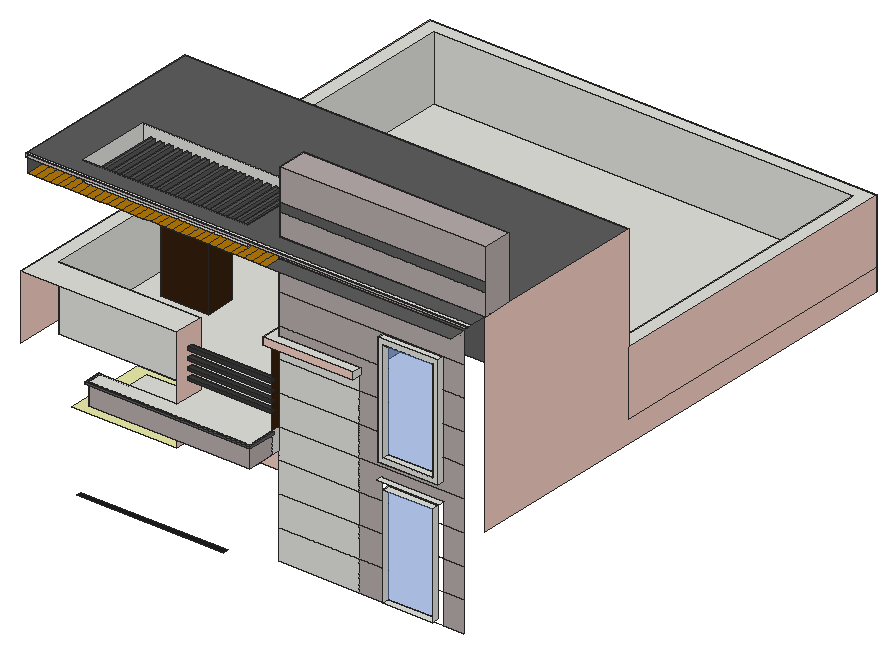
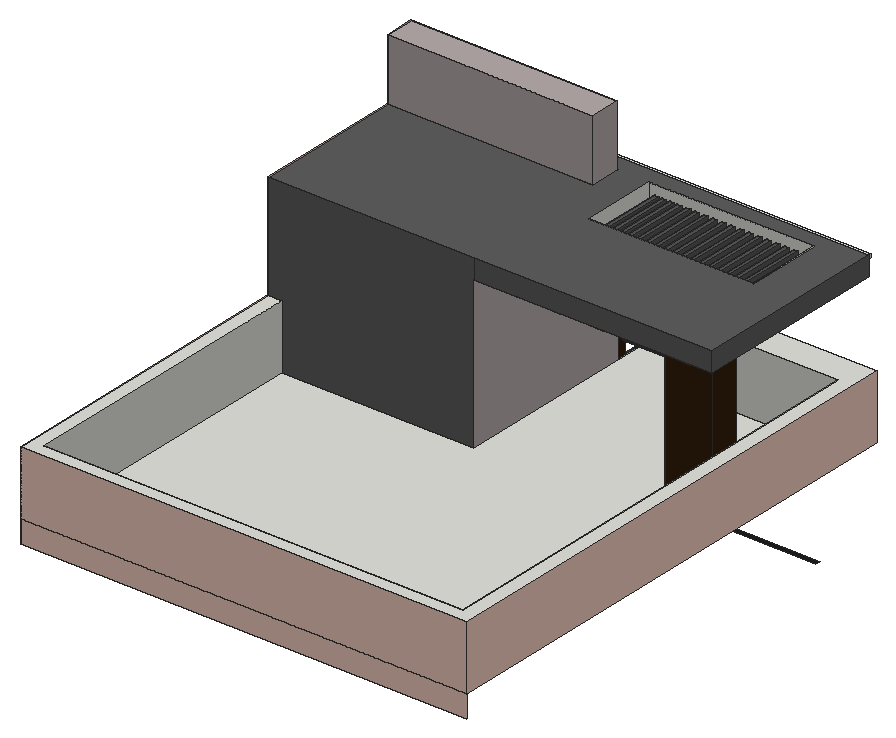
# SketchUp Ruby script. Lengths in inches.
U = 1.inch
M = Sketchup.active_model
def pt(a) = Geom::Point3d.new(a.map { |v| v * U })
def face(e, loops, mat)
  f = e.add_face(loops[0].map { |a| pt(a) })
  loops[1..].each { |l| e.add_face(l.map { |a| pt(a) }).erase! }
  f.material = f.back_material = mat if mat
  f
end
# faces: each face lists its corners as indices into pts; further lists are holes
def faces(e, pts, list, mat = nil) = list.each { |f| face(e, (f[0].is_a?(Array) ? f : [f]).map { |l| l.map { |i| pts[i] } }, mat) }
# xy, xz, yz: faces in a plane at the given z, y or x. An outline is a flat list of corners, or four numbers for a rectangle; further outlines are holes
def ring(l) = l.size == 4 ? [[l[0], l[1]], [l[2], l[1]], [l[2], l[3]], [l[0], l[3]]] : l.each_slice(2).to_a
def flat(e, list, mat, &to3) = list.each { |f| face(e, (f[0].is_a?(Array) ? f : [f]).map { |l| ring(l).map { |u, v| to3.(u, v) } }, mat) }
def xy(e, z, list, mat = nil) = flat(e, list, mat) { |x, y| [x, y, z] }
def xz(e, y, list, mat = nil) = flat(e, list, mat) { |x, z| [x, y, z] }
def yz(e, x, list, mat = nil) = flat(e, list, mat) { |y, z| [x, y, z] }
def lines(e, pts, list) = list.each { |a, b| e.add_line(pt(pts[a]), pt(pts[b])) }
# prism: a flat outline (further loops are holes) pulled along v
def prism(e, loops, v, mat = nil)
  f = face(e, loops, mat); d = Geom::Vector3d.new(v.map { |x| x * U })
  f.pushpull(f.normal.samedirection?(d) ? d.length : -d.length)
end
def box(e, o, s, mat = nil) = prism(e, [[o, [o[0] + s[0], o[1], o[2]], [o[0] + s[0], o[1] + s[1], o[2]], [o[0], o[1] + s[1], o[2]]]], [0, 0, s[2]], mat)
def at(x, y, z, deg = 0) = Geom::Transformation.translation(pt([x, y, z])) * Geom::Transformation.rotation(ORIGIN, Z_AXIS, deg.degrees)
def axes(o, x, y, z) = Geom::Transformation.new([*x, 0, *y, 0, *z, 0, *pt(o).to_a, 1])
def part(name) = M.definitions.add(name)
# library, detail: a bought-in or finely detailed component or shape, given as its bounding box
def library(name, o, s) = part(name).tap { |d| box(d.entities, o, s) }
def detail(e, o, s) = box(e.add_group.entities, o, s)
def put(e, d, t, mat = nil) = e.add_instance(d, t).tap { |i| i.material = mat if mat }
def group(e, t, mat = nil) = e.add_group.tap { |g| g.transformation = t; g.material = mat if mat }.entities
root = M.entities
M.materials.add("Generic").color = [94, 94, 94]
M.materials.add("Generic\#1").color = [182, 171, 171]
M.materials.add("Generic\#4").color = [178, 120, 8]
M.materials.add("Generic\#5").color = [242, 205, 193]
M.materials.add("Generic\#7").color = [235, 237, 171]
M.materials.add("[Color M06]").color = [86, 86, 86]
M.materials.add("[Color M07]").color = [58, 58, 58]
M.materials.add("[Color M08]").color = [30, 30, 30]
M.materials.add("[Translucent Glass Blue]").color = [100, 149, 237]
M.materials["[Translucent Glass Blue]"].alpha = 0.5
M.materials.add("[Wood Floor Dark]").color = [53, 32, 13]
xy(root,173.625,[[43.84,66.48,170.12,70.85]],"[Color M08]")
xy(root,177.11,[[299.95,74.6,342.64,79.98]])
xy(root,217.95,[[81.41,131.85,161.72,167.54]])
xy(root,243.9375,[[43.84,60.73,133.85,79.98],[43.84,79.98,206.39,131.85]],"Generic\#7")
xy(root,258.75,[[170.12,61.18,206.39,72.04]])
xy(root,258.75,[[68.34,48.23,68.34,60.73,133.85,60.73,170.12,61.18,206.39,61.18,206.39,48.23]],"Generic\#1")
xy(root,258.75,[[133.85,60.73,133.85,79.98,206.39,79.98,206.39,72.04,170.12,72.04,170.12,61.18]],"Generic\#5")
xy(root,264.3,[[299.95,74.6,342.64,79.98]])
xy(root,269.6,[[294.65,74.6,347.95,79.98]])
xy(root,275.5,[[66.59,46.29,66.59,61.66,68.34,61.66,68.34,48.23,206.39,48.23,206.39,71.98,208.2,71.98,208.2,46.29]],"Generic")
xy(root,277.5,[[[68.34,48.23,206.39,48.23,206.39,234.29,371.3125,234.29,371.3125,488.54,12.4375,488.54,12.4375,86.6,133.91,86.6,133.91,60.73,68.34,60.73],[32.8,169.87,74.12,194.99]],[93.09,60.73,133.91,79.98]])
xy(root,277.5,[[66.59,46.29,208.2,46.29,208.2,71.98,206.39,71.98,206.39,48.23,68.34,48.23,68.34,61.66,66.59,61.66]],"Generic")
xy(root,284.35,[[295.76,74.6,346.84,79.98]])
xy(root,288.55,[[299.95,74.6,342.64,79.98]])
xy(root,290.9,[[133.91,72.1,206.39,75.91]],"[Color M07]")
xy(root,293.86,[[133.91,72.1,206.39,75.91]],"[Color M07]")
xy(root,298.59,[[133.91,72.1,206.39,75.91]],"[Color M07]")
xy(root,301.54,[[133.91,72.1,206.39,75.91]],"[Color M07]")
xy(root,306.28,[[133.91,72.1,206.39,75.91]],"[Color M07]")
xy(root,309.23,[[133.91,72.1,206.39,75.91]],"[Color M07]")
xy(root,313.96,[[133.91,72.1,206.39,75.91]],"[Color M07]")
xy(root,317.11,[[133.91,72.1,206.39,75.91]],"[Color M07]")
xy(root,332.8125,[[0,60.73,133.91,60.73,133.91,86.6,12.4375,86.6,12.4375,488.54,371.3125,488.54,371.3125,234.29,382.6875,234.29,382.6875,499.98,0,499.98]])
xy(root,341.34,[[199.14,71.98,206.39,127.29],[206.39,71.98,274.66,79.98],[274.66,71.98,276.22,79.98]])
xy(root,347.28,[[199.14,71.98,276.22,71.98,276.22,79.98,206.39,79.98,206.39,127.29,199.14,127.29]])
xy(root,375.73,[[299.95,74.6,342.64,79.98]])
xy(root,379.93,[[295.76,74.6,346.84,79.98]])
xy(root,406.6875,[[2.375,65.66,2.5,234.29]])
xy(root,406.6875,[[206.39,65.66,365.0625,79.98]],"Generic")
xy(root,406.6875,[[2.5,65.66,8.69,234.29],[8.69,65.66,14.88,234.29],[14.88,65.66,21.07,234.29],[21.07,65.66,27.25,234.29],[27.25,65.66,33.44,234.29],
  [33.44,65.66,33.44,234.29,39.63,234.29,39.63,144.39,38.29,144.39,38.29,79.45,39.63,79.45,39.63,65.66],[39.63,65.66,45.82,79.45],[45.82,65.66,52,79.45],[52,65.66,58.19,79.45],[58.19,65.66,64.38,79.45],
  [64.38,65.66,70.57,79.45],[70.57,65.66,76.75,79.45],[76.75,65.66,82.94,79.45],[82.94,65.66,89.13,79.45],[89.13,65.66,95.32,79.45],
  [95.32,65.66,101.5,79.45],[101.5,65.66,107.69,79.45],[107.69,65.66,113.88,79.45],[113.88,65.66,120.07,79.45],[120.07,65.66,126.25,79.45],
  [126.25,65.66,132.44,79.45],[132.44,65.66,138.63,79.45],[138.63,65.66,144.82,79.45],[144.82,65.66,151,79.45],[151,65.66,157.19,79.45],
  [157.19,65.66,163.38,79.45],[163.38,65.66,169.57,79.45],[169.57,65.66,175.75,79.45],[175.75,65.66,175.75,79.45,179.85,79.45,179.85,144.39,175.75,144.39,175.75,234.29,181.94,234.29,181.94,65.66],[181.94,65.66,188.13,234.29],
  [188.13,65.66,194.32,234.29],[194.32,65.66,200.5,234.29],[200.5,65.66,206.39,234.29],[39.63,144.39,45.82,234.29],[45.82,144.39,52,234.29],
  [52,144.39,58.19,234.29],[58.19,144.39,64.38,234.29],[64.38,144.39,70.57,234.29],[70.57,144.39,76.75,234.29],[76.75,144.39,82.94,234.29],
  [82.94,144.39,89.13,234.29],[89.13,144.39,95.32,234.29],[95.32,144.39,101.5,234.29],[101.5,144.39,107.69,234.29],[107.69,144.39,113.88,234.29],
  [113.88,144.39,120.07,234.29],[120.07,144.39,126.25,234.29],[126.25,144.39,132.44,234.29],[132.44,144.39,138.63,234.29],[138.63,144.39,144.82,234.29],
  [144.82,144.39,151,234.29],[151,144.39,157.19,234.29],[157.19,144.39,163.38,234.29],[163.38,144.39,169.57,234.29],[169.57,144.39,175.75,234.29]],"Generic\#4")
xy(root,409.0625,[[44.89,79.45,48.46,144.39],[52.58,79.45,56.14,144.39],[60.27,79.45,63.83,144.39],[67.96,79.45,71.52,144.39],[75.64,79.45,79.21,144.39],
  [83.33,79.45,86.89,144.39],[91.02,79.45,94.58,144.39],[98.71,79.45,102.27,144.39],[106.39,79.45,109.96,144.39],[114.02,79.45,117.58,144.39],
  [121.64,79.45,125.21,144.39],[129.27,79.45,132.83,144.39],[136.89,79.45,140.46,144.39],[144.52,79.45,148.08,144.39],[152.14,79.45,155.71,144.39],
  [158.71,79.45,162.27,144.39],[165.27,79.45,168.83,144.39],[171.83,79.45,175.39,144.39]],"[Color M06]")
xy(root,409.5625,[[32.8,169.87,74.12,194.99]])
xy(root,414.625,[[44.89,79.45,48.46,144.39],[52.58,79.45,56.14,144.39],[60.27,79.45,63.83,144.39],[67.96,79.45,71.52,144.39],[75.64,79.45,79.21,144.39],
  [83.33,79.45,86.89,144.39],[91.02,79.45,94.58,144.39],[98.71,79.45,102.27,144.39],[106.39,79.45,109.96,144.39],[114.02,79.45,117.58,144.39],
  [121.64,79.45,125.21,144.39],[129.27,79.45,132.83,144.39],[136.89,79.45,140.46,144.39],[144.52,79.45,148.08,144.39],[152.14,79.45,155.71,144.39],
  [158.71,79.45,162.27,144.39],[165.27,79.45,168.83,144.39],[171.83,79.45,175.39,144.39]],"[Color M06]")
xy(root,420.375,[[2.375,63.6,379.5625,65.66]],"Generic\#1")
xy(root,423.375,[[2.375,63.6,382.6875,65.66],[206.39,79.98,382.6875,80.85],[206.39,80.85,382.6875,106.29]])
xy(root,423.375,[[[2.375,65.66,382.6875,65.66,382.6875,79.98,206.39,79.98,206.39,106.29,382.6875,106.29,382.6875,234.29,2.375,234.29],[38.29,79.45,179.85,144.39]]],"Generic")
xy(root,476.625,[[206.39,80.85,382.6875,106.29]],"Generic\#1")
xz(root,46.29,[[66.59,275.5,208.2,277.5]],"Generic")
xz(root,48.23,[[68.34,275.5,206.39,277.5]])
xz(root,48.23,[[68.34,258.75,206.39,275.5]],"Generic\#1")
xz(root,60.73,[[68.34,258.75,93.09,277.5]])
xz(root,61.66,[[66.59,275.5,68.34,277.5]])
xz(root,71.98,[[199.14,341.34,276.22,347.28]],"Generic\#5")
xz(root,72.1,[[133.91,290.9,206.39,293.86],[133.91,298.59,206.39,301.54],[133.91,306.28,206.39,309.23],[133.91,313.96,206.39,317.11]],"[Color M07]")
xz(root,74.6,[[[295.76,284.35,346.84,379.93],[299.95,288.55,342.64,375.73]]])
xz(root,75.91,[[133.91,290.9,206.39,293.86],[133.91,298.59,206.39,301.54],[133.91,306.28,206.39,309.23],[133.91,313.96,206.39,317.11]],"[Color M07]")
xz(root,79.45,[[[38.29,406.6875,179.85,423.375],[44.89,409.0625,48.46,414.625],[52.58,409.0625,56.14,414.625],[60.27,409.0625,63.83,414.625],[67.96,409.0625,71.52,414.625],[75.64,409.0625,79.21,414.625],[83.33,409.0625,86.89,414.625],[91.02,409.0625,94.58,414.625],[98.71,409.0625,102.27,414.625],[106.39,409.0625,109.96,414.625],[114.02,409.0625,117.58,414.625],[121.64,409.0625,125.21,414.625],[129.27,409.0625,132.83,414.625],[136.89,409.0625,140.46,414.625],[144.52,409.0625,148.08,414.625],[152.14,409.0625,155.71,414.625],[158.71,409.0625,162.27,414.625],[165.27,409.0625,168.83,414.625],[171.83,409.0625,175.39,414.625]]])
xz(root,79.98,[[206.39,173.95,274.66,199.81],[206.39,199.81,274.66,225.67],[206.39,225.67,274.66,251.53],[206.39,251.53,274.66,277.39],[206.39,277.39,274.66,303.25],
  [206.39,303.25,274.66,329.11],[206.39,329.11,274.66,341.34],[206.39,341.34,276.22,347.28]])
xz(root,79.98,[[274.66,173.95,294.65,199.81],[347.95,173.95,365.0625,199.81],[274.66,199.81,294.65,225.67],[347.95,199.81,365.0625,225.67],[274.66,225.67,294.65,251.53],
  [347.95,225.67,365.0625,251.53],[274.66,251.53,294.65,251.53,294.65,269.6,347.95,269.6,347.95,251.53,365.0625,251.53,365.0625,277.39,274.66,277.39],[274.66,277.39,365.0625,277.39,365.0625,303.25,346.84,303.25,346.84,284.35,295.76,284.35,295.76,303.25,274.66,303.25],[274.66,303.25,295.76,329.11],[346.84,303.25,365.0625,329.11],
  [274.66,329.11,295.76,329.11,295.76,354.97,206.39,354.97,206.39,347.28,276.22,347.28,276.22,341.34,274.66,341.34],[346.84,329.11,365.0625,354.97],[206.39,354.97,295.76,354.97,295.76,379.93,346.84,379.93,346.84,354.97,365.0625,354.97,365.0625,380.83,206.39,380.83],[206.39,380.83,365.0625,406.6875]],"Generic\#1")
xz(root,79.98,[[133.85,243.9375,206.39,258.75]],"Generic\#5")
xz(root,79.98,[[299.95,177.11,342.64,264.3],[299.95,288.55,342.64,375.73]],"[Translucent Glass Blue]")
xz(root,80.85,[[206.39,441.75,382.6875,449.75]],"Generic")
xz(root,80.85,[[206.39,423.375,382.6875,441.75],[206.39,449.75,382.6875,476.625]],"Generic\#1")
xz(root,86.6,[[12.4375,277.5,133.91,332.8125]])
xz(root,106.29,[[206.39,423.375,382.6875,476.625]],"Generic\#1")
xz(root,127.29,[[199.14,341.34,206.39,347.28]])
xz(root,144.39,[[[38.29,406.6875,179.85,423.375],[44.89,409.0625,48.46,414.625],[52.58,409.0625,56.14,414.625],[60.27,409.0625,63.83,414.625],[67.96,409.0625,71.52,414.625],[75.64,409.0625,79.21,414.625],[83.33,409.0625,86.89,414.625],[91.02,409.0625,94.58,414.625],[98.71,409.0625,102.27,414.625],[106.39,409.0625,109.96,414.625],[114.02,409.0625,117.58,414.625],[121.64,409.0625,125.21,414.625],[129.27,409.0625,132.83,414.625],[136.89,409.0625,140.46,414.625],[144.52,409.0625,148.08,414.625],[152.14,409.0625,155.71,414.625],[158.71,409.0625,162.27,414.625],[165.27,409.0625,168.83,414.625],[171.83,409.0625,175.39,414.625]]])
xz(root,169.87,[[32.8,277.5,74.12,409.5625]],"[Wood Floor Dark]")
xz(root,194.99,[[32.8,277.5,74.12,409.5625]],"[Wood Floor Dark]")
xz(root,234.29,[[206.39,277.5,206.39,423.375,382.6875,423.375,382.6875,332.8125,371.3125,332.8125,371.3125,277.5],[2.375,406.6875,206.39,423.375]],"Generic")
xz(root,488.54,[[12.4375,277.5,371.3125,332.8125]])
xz(root,499.98,[[0,258.75,382.6875,277.5],[0,277.5,382.6875,332.8125]],"Generic\#5")
yz(root,0,[[60.73,277.5,499.98,332.8125]],"Generic\#5")
yz(root,2.375,[[63.6,420.375,65.66,423.375]])
yz(root,2.375,[[65.66,406.6875,234.29,423.375]],"Generic")
yz(root,12.4375,[[86.6,277.5,488.54,332.8125]])
yz(root,32.8,[[169.87,277.5,194.99,409.5625]],"[Wood Floor Dark]")
yz(root,38.29,[[79.45,406.6875,144.39,423.375]])
yz(root,44.89,[[79.45,409.0625,144.39,414.625]],"[Color M06]")
yz(root,48.46,[[79.45,409.0625,144.39,414.625]],"[Color M06]")
yz(root,52.58,[[79.45,409.0625,144.39,414.625]],"[Color M06]")
yz(root,56.14,[[79.45,409.0625,144.39,414.625]],"[Color M06]")
yz(root,60.27,[[79.45,409.0625,144.39,414.625]],"[Color M06]")
yz(root,63.83,[[79.45,409.0625,144.39,414.625]],"[Color M06]")
yz(root,66.59,[[46.29,275.5,61.66,277.5]],"Generic")
yz(root,67.96,[[79.45,409.0625,144.39,414.625]],"[Color M06]")
yz(root,68.34,[[48.23,275.5,60.73,277.5],[60.73,275.5,61.66,277.5]])
yz(root,68.34,[[48.23,258.75,60.73,275.5]],"Generic\#1")
yz(root,71.52,[[79.45,409.0625,144.39,414.625]],"[Color M06]")
yz(root,74.12,[[169.87,277.5,194.99,409.5625]],"[Wood Floor Dark]")
yz(root,75.64,[[79.45,409.0625,144.39,414.625]],"[Color M06]")
yz(root,79.21,[[79.45,409.0625,144.39,414.625]],"[Color M06]")
yz(root,83.33,[[79.45,409.0625,144.39,414.625]],"[Color M06]")
yz(root,86.89,[[79.45,409.0625,144.39,414.625]],"[Color M06]")
yz(root,91.02,[[79.45,409.0625,144.39,414.625]],"[Color M06]")
yz(root,94.58,[[79.45,409.0625,144.39,414.625]],"[Color M06]")
yz(root,98.71,[[79.45,409.0625,144.39,414.625]],"[Color M06]")
yz(root,102.27,[[79.45,409.0625,144.39,414.625]],"[Color M06]")
yz(root,106.39,[[79.45,409.0625,144.39,414.625]],"[Color M06]")
yz(root,109.96,[[79.45,409.0625,144.39,414.625]],"[Color M06]")
yz(root,114.02,[[79.45,409.0625,144.39,414.625]],"[Color M06]")
yz(root,117.58,[[79.45,409.0625,144.39,414.625]],"[Color M06]")
yz(root,121.64,[[79.45,409.0625,144.39,414.625]],"[Color M06]")
yz(root,125.21,[[79.45,409.0625,144.39,414.625]],"[Color M06]")
yz(root,129.27,[[79.45,409.0625,144.39,414.625]],"[Color M06]")
yz(root,132.83,[[79.45,409.0625,144.39,414.625]],"[Color M06]")
yz(root,133.85,[[60.73,243.9375,79.98,258.75]],"Generic\#5")
yz(root,133.91,[[[60.73,277.5,86.6,332.8125],[72.1,313.96,75.91,317.11],[72.1,306.28,75.91,309.23],[72.1,298.59,75.91,301.54],[72.1,290.9,75.91,293.86]]],"Generic\#5")
yz(root,136.89,[[79.45,409.0625,144.39,414.625]],"[Color M06]")
yz(root,140.46,[[79.45,409.0625,144.39,414.625]],"[Color M06]")
yz(root,144.52,[[79.45,409.0625,144.39,414.625]],"[Color M06]")
yz(root,148.08,[[79.45,409.0625,144.39,414.625]],"[Color M06]")
yz(root,152.14,[[79.45,409.0625,144.39,414.625]],"[Color M06]")
yz(root,155.71,[[79.45,409.0625,144.39,414.625]],"[Color M06]")
yz(root,158.71,[[79.45,409.0625,144.39,414.625]],"[Color M06]")
yz(root,162.27,[[79.45,409.0625,144.39,414.625]],"[Color M06]")
yz(root,165.27,[[79.45,409.0625,144.39,414.625]],"[Color M06]")
yz(root,168.83,[[79.45,409.0625,144.39,414.625]],"[Color M06]")
yz(root,171.83,[[79.45,409.0625,144.39,414.625]],"[Color M06]")
yz(root,175.39,[[79.45,409.0625,144.39,414.625]],"[Color M06]")
yz(root,179.85,[[79.45,406.6875,144.39,423.375]])
yz(root,199.14,[[71.98,341.34,127.29,347.28]],"Generic\#5")
yz(root,206.39,[[71.98,258.75,79.98,277.5],[48.23,275.5,71.98,277.5],[79.98,341.34,127.29,347.28]])
yz(root,206.39,[[48.23,258.75,71.98,275.5],[79.98,277.5,79.98,341.34,127.29,341.34,127.29,347.28,79.98,347.28,79.98,406.6875,234.29,406.6875,234.29,277.5],[80.85,423.375,106.29,476.625]],"Generic\#1")
yz(root,206.39,[[[71.98,277.5,79.98,341.34],[72.1,313.96,75.91,317.11],[72.1,306.28,75.91,309.23],[72.1,298.59,75.91,301.54],[72.1,290.9,75.91,293.86]]],"[Wood Floor Dark]")
yz(root,208.2,[[46.29,275.5,71.98,277.5]],"Generic")
yz(root,276.22,[[71.98,341.34,79.98,347.28]])
yz(root,295.76,[[74.6,284.35,79.98,379.93]])
yz(root,299.95,[[74.6,177.11,79.98,264.3],[74.6,288.55,79.98,375.73]])
yz(root,342.64,[[74.6,177.11,79.98,264.3],[74.6,288.55,79.98,375.73]])
yz(root,346.84,[[74.6,284.35,79.98,379.93]])
yz(root,371.3125,[[234.29,277.5,488.54,332.8125]])
yz(root,382.6875,[[80.85,423.375,106.29,476.625]],"Generic\#1")
yz(root,382.6875,[[79.98,258.75,499.98,258.75,499.98,277.5,234.29,277.5,234.29,423.375,79.98,423.375],[234.29,277.5,499.98,332.8125]],"Generic\#5")
p = [[93.09,79.98,258.75],[93.09,79.98,277.5],[371.1875,65.66,412.43],[371.1875,65.66,412.39],[373.6875,65.66,412.43],[373.6875,65.66,412.39],
  [295.76,79.98,354.97],[299.95,79.98,354.97],[342.64,79.98,354.97],[346.84,79.98,354.97],[295.76,79.98,329.11],[299.95,79.98,329.11],
  [342.64,79.98,329.11],[346.84,79.98,329.11],[295.76,79.98,303.25],[299.95,79.98,303.25],[342.64,79.98,303.25],[346.84,79.98,303.25],
  [294.65,79.98,251.53],[299.95,79.98,251.53],[342.64,79.98,251.53],[347.95,79.98,251.53],[294.65,79.98,225.67],[299.95,79.98,225.67],
  [342.64,79.98,225.67],[347.95,79.98,225.67],[294.65,79.98,199.81],[299.95,79.98,199.81],[342.64,79.98,199.81],[347.95,79.98,199.81],
  [294.65,79.98,173.95],[347.95,79.98,173.95],[133.85,79.98,258.75]]
lines(root,p,[[0,1],[2,3],[4,5],[6,7],[8,9],[10,11],[12,13],[14,15],[16,17],[18,19],[20,21],[22,23],
  [24,25],[26,27],[28,29],[30,31],[0,32]])
